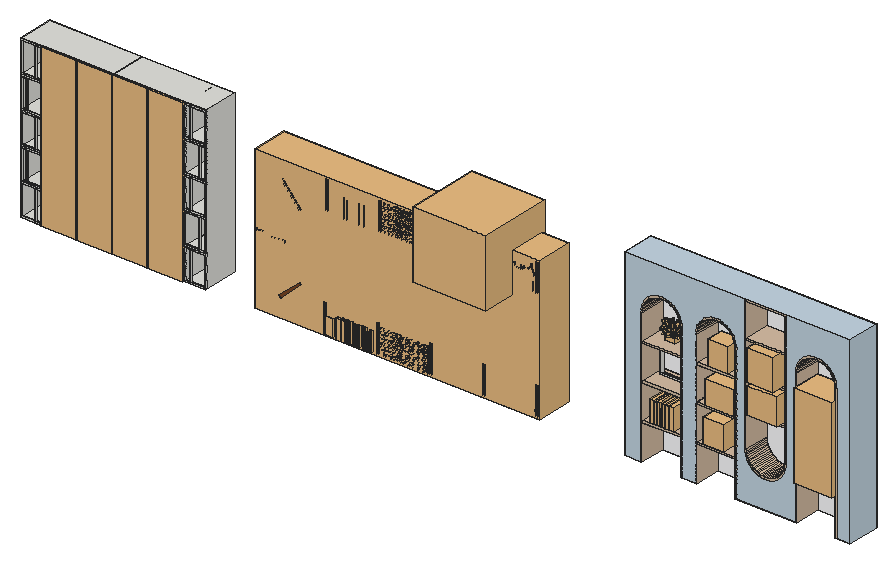
# SketchUp Ruby script. Lengths in millimetres.
U = 1.mm
M = Sketchup.active_model
def pt(a) = Geom::Point3d.new(a.map { |v| v * U })
def face(e, loops, mat)
  f = e.add_face(loops[0].map { |a| pt(a) })
  loops[1..].each { |l| e.add_face(l.map { |a| pt(a) }).erase! }
  f.material = f.back_material = mat if mat
  f
end
# faces: each face lists its corners as indices into pts; further lists are holes
def faces(e, pts, list, mat = nil) = list.each { |f| face(e, (f[0].is_a?(Array) ? f : [f]).map { |l| l.map { |i| pts[i] } }, mat) }
# xy, xz, yz: faces in a plane at the given z, y or x. An outline is a flat list of corners, or four numbers for a rectangle; further outlines are holes
def ring(l) = l.size == 4 ? [[l[0], l[1]], [l[2], l[1]], [l[2], l[3]], [l[0], l[3]]] : l.each_slice(2).to_a
def flat(e, list, mat, &to3) = list.each { |f| face(e, (f[0].is_a?(Array) ? f : [f]).map { |l| ring(l).map { |u, v| to3.(u, v) } }, mat) }
def xy(e, z, list, mat = nil) = flat(e, list, mat) { |x, y| [x, y, z] }
def xz(e, y, list, mat = nil) = flat(e, list, mat) { |x, z| [x, y, z] }
def yz(e, x, list, mat = nil) = flat(e, list, mat) { |y, z| [x, y, z] }
def lines(e, pts, list) = list.each { |a, b| e.add_line(pt(pts[a]), pt(pts[b])) }
# prism: a flat outline (further loops are holes) pulled along v
def prism(e, loops, v, mat = nil)
  f = face(e, loops, mat); d = Geom::Vector3d.new(v.map { |x| x * U })
  f.pushpull(f.normal.samedirection?(d) ? d.length : -d.length)
end
def box(e, o, s, mat = nil) = prism(e, [[o, [o[0] + s[0], o[1], o[2]], [o[0] + s[0], o[1] + s[1], o[2]], [o[0], o[1] + s[1], o[2]]]], [0, 0, s[2]], mat)
def at(x, y, z, deg = 0) = Geom::Transformation.translation(pt([x, y, z])) * Geom::Transformation.rotation(ORIGIN, Z_AXIS, deg.degrees)
def axes(o, x, y, z) = Geom::Transformation.new([*x, 0, *y, 0, *z, 0, *pt(o).to_a, 1])
def part(name) = M.definitions.add(name)
# library, detail: a bought-in or finely detailed component or shape, given as its bounding box
def library(name, o, s) = part(name).tap { |d| box(d.entities, o, s) }
def detail(e, o, s) = box(e.add_group.entities, o, s)
def put(e, d, t, mat = nil) = e.add_instance(d, t).tap { |i| i.material = mat if mat }
def group(e, t, mat = nil) = e.add_group.tap { |g| g.transformation = t; g.material = mat if mat }.entities
root = M.entities
M.materials.add("Material~26").color = [121, 120, 117]
M.materials.add("Material~27").color = [130, 129, 127]
M.materials.add("Material~28").color = [131, 130, 129]
M.materials.add("Material~29").color = [119, 120, 115]
M.materials.add("Material~30").color = [120, 117, 114]
M.materials.add("Material~31").color = [121, 119, 117]
M.materials.add("Material~32").color = [21, 20, 18]
M.materials.add("Material~33").color = [25, 25, 23]
M.materials.add("Material~34").color = [109, 108, 106]
M.materials.add("Material~35").color = [120, 119, 118]
M.materials.add("Material~36").color = [34, 33, 33]
M.materials.add("Material~37").color = [104, 103, 91]
M.materials.add("Material~38").color = [106, 95, 72]
M.materials.add("Material~39").color = [33, 29, 24]
M.materials.add("Material~40").color = [127, 124, 119]
M.materials.add("Material~41").color = [118, 115, 112]
M.materials.add("Material~42").color = [32, 34, 33]
M.materials.add("Material~43").color = [40, 35, 29]
M.materials.add("Material~44").color = [125, 125, 122]
M.materials.add("Material~45").color = [118, 122, 122]
M.materials.add("Material~46").color = [30, 29, 26]
M.materials.add("Material~47").color = [27, 28, 21]
M.materials.add("Material~48").color = [21, 20, 18]
M.materials.add("Material~49").color = [127, 124, 121]
M.materials.add("Material~50").color = [128, 121, 110]
M.materials.add("Material~51").color = [124, 124, 122]
M.materials.add("Material~52").color = [71, 70, 67]
M.materials.add("Material~53").color = [25, 26, 25]
M.materials.add("Material~54").color = [122, 115, 107]
M.materials.add("Material~55").color = [102, 101, 100]
M.materials.add("Material~56").color = [120, 119, 118]
M.materials.add("Material~57").color = [109, 108, 106]
M.materials.add("Material~58").color = [104, 103, 91]
M.materials.add("Material~59").color = [106, 95, 72]
M.materials.add("PDM_Timber_01").color = [134, 117, 87]
M.materials.add("[Blinds_Vertical_Stripe_Gray]").color = [159, 159, 159]
M.materials.add("[Color M09]").color = [0, 0, 0]
M.materials.add("[Color_001]").color = [226, 226, 226]
M.materials.add("[Color_006]").color = [86, 86, 86]
M.materials.add("[Color_A05]").color = [255, 204, 204]
M.materials.add("[Color_A19]").color = [102, 61, 61]
M.materials.add("[Color_A20]").color = [102, 81, 81]
M.materials.add("[Color_B03]").color = [255, 140, 101]
M.materials.add("[Color_B04]").color = [255, 178, 153]
M.materials.add("[Color_B05]").color = [255, 216, 204]
M.materials.add("[Color_C05]").color = [255, 229, 204]
M.materials.add("[Color_C15]").color = [153, 137, 122]
M.materials.add("[Color_D05]").color = [255, 242, 204]
M.materials.add("[Color_D10]").color = [204, 193, 163]
M.materials.add("[Color_D20]").color = [102, 96, 81]
M.materials.add("[Color_E04]").color = [255, 255, 153]
M.materials.add("[Color_E05]").color = [255, 255, 204]
M.materials.add("[Color_E18]").color = [102, 102, 40]
M.materials.add("[Color_G15]").color = [122, 153, 122]
M.materials.add("[Color_I10]").color = [163, 163, 204]
M.materials.add("[Color_I13]").color = [61, 61, 153]
M.materials.add("[Color_I22]").color = [10, 10, 51]
M.materials.add("[Color_L04]").color = [255, 153, 204]
M.materials.add("[Formica Laminate Light]").color = [213, 189, 164]
M.materials.add("[Metal_Brass_Ceiling]").color = [125, 102, 93]
M.materials.add("[Polished Concrete New]").color = [168, 168, 168]
M.materials.add("[Quartz Light Grey]").color = [251, 251, 252]
M.materials.add("[Terrazzo Light Blue]").color = [196, 214, 227]
M.materials.add("[Wood Veneer 01]").color = [120, 70, 37]
c1 = part("Rectangular frame")
prism(c1.entities,[[[300,0,450],[0,0,450],[0,0,0],[300,0,0]],[[284,0,16],[99.2,0,16],[99.2,0,434],[284,0,434]],[[80.7,0,434],[80.7,0,16],[16,0,16],[16,0,434]]],[0,16,0])
c2 = part("Joinery panel")
box(c2.entities,[0,0,0],[30,500,390])
c3 = part("Row of books \#2")
xy(c3.entities,211.6,[[0,541.4,180.2,552.7]],"[Color_D05]")
xy(c3.entities,221.1,[[0,502,180.2,541.4]],"[Color_L04]")
xy(c3.entities,226,[[0,211.2,180.2,238.8]],"[Color_A20]")
xy(c3.entities,226,[[0,179,180.2,194.7]],"[Color_E05]")
xy(c3.entities,229.1,[[0,146.8,180.2,158.7],[0,194.7,180.2,211.2]],"[Color_I10]")
xy(c3.entities,230.9,[[0,552.7,180.2,581.8]],"[Color_C05]")
xy(c3.entities,239.2,[[0,238.8,180.2,259.8]],"[Color_B03]")
xy(c3.entities,246.4,[[0,0,180.2,14.4]],"[Color_I13]")
xy(c3.entities,247,[[0,115.8,180.2,122.7]],"[Color_A05]")
xy(c3.entities,257.4,[[0,438.1,180.2,454.4]],"[Color_C05]")
xy(c3.entities,259.7,[[0,489.2,180.2,502]],"[Color_E18]")
xy(c3.entities,262,[[0,122.7,180.2,132.4]],"[Color_A05]")
xy(c3.entities,262.3,[[0,72.3,180.2,83.9]],"[Color_B05]")
xy(c3.entities,267.7,[[0,278.8,180.2,301.7]],"[Color_006]")
xy(c3.entities,274.4,[[0,104.2,180.2,115.8]],"[Color_001]")
xy(c3.entities,274.4,[[0,83.9,180.2,104.2]],"[Color_A19]")
xy(c3.entities,274.9,[[0,158.7,180.2,179]],"[Color_D05]")
xy(c3.entities,275.5,[[0,395.3,180.2,438.1]],"[Color_B05]")
xy(c3.entities,275.5,[[0,339.9,180.2,357.7]],"[Color_D10]")
xy(c3.entities,275.5,[[0,259.8,180.2,278.8]],"[Color_E05]")
xy(c3.entities,277.8,[[0,14.4,180.2,23.5]],"[Color_E05]")
xy(c3.entities,278.7,[[0,301.7,180.2,315.8]],"[Color_B04]")
xy(c3.entities,278.7,[[0,357.7,180.2,375.2]],"[Color_E04]")
xy(c3.entities,282.4,[[0,59.1,180.2,72.3]],"[Color_B05]")
xy(c3.entities,283.3,[[0,315.8,180.2,339.9]],"[Color_006]")
xy(c3.entities,283.3,[[0,375.2,180.2,395.3]],"[Color_C15]")
xy(c3.entities,298.5,[[0,132.4,180.2,146.8]],"[Color_E05]")
xy(c3.entities,300,[[0,44.1,180.2,59.1]],"[Color_G15]")
xy(c3.entities,304,[[0,454.4,180.2,466.9]],"[Color_C05]")
xy(c3.entities,332.2,[[0,466.9,180.2,489.2]],"[Color_C05]")
xy(c3.entities,342,[[0,23.5,180.2,44.1]],"[Color_006]")
xz(c3.entities,14.4,[[0,246.4,180.2,277.8]],"[Color_E05]")
xz(c3.entities,23.5,[[0,277.8,180.2,342]],"[Color_D20]")
xz(c3.entities,44.1,[[0,300,180.2,342]],"[Color_006]")
xz(c3.entities,59.1,[[0,282.4,180.2,300]],"[Color_G15]")
xz(c3.entities,72.3,[[0,262.3,180.2,282.4]],"[Color_B05]")
xz(c3.entities,83.9,[[0,262.3,180.2,274.4]],"[Metal_Brass_Ceiling]")
xz(c3.entities,115.8,[[0,247,180.2,274.4]],"[Metal_Brass_Ceiling]")
xz(c3.entities,122.7,[[0,247,180.2,262]],"[Metal_Brass_Ceiling]")
xz(c3.entities,132.4,[[0,262,180.2,298.5]],"[Metal_Brass_Ceiling]")
xz(c3.entities,146.8,[[0,229.1,180.2,298.5]],"[Color_E05]")
xz(c3.entities,158.7,[[0,229.1,180.2,274.9]],"[Metal_Brass_Ceiling]")
xz(c3.entities,179,[[0,226,180.2,274.9]],"[Color_D05]")
xz(c3.entities,194.7,[[0,226,180.2,229.1]],"[Metal_Brass_Ceiling]")
xz(c3.entities,211.2,[[0,226,180.2,229.1]],"[Metal_Brass_Ceiling]")
xz(c3.entities,238.8,[[0,226,180.2,239.2]],"[Color_B03]")
xz(c3.entities,259.8,[[0,239.2,180.2,275.5]],"[Color_E05]")
xz(c3.entities,278.8,[[0,267.7,180.2,275.5]],"[Metal_Brass_Ceiling]")
xz(c3.entities,301.7,[[0,267.7,180.2,278.7]],"[Color_B04]")
xz(c3.entities,315.8,[[0,278.7,180.2,283.3]],"[Color_006]")
xz(c3.entities,339.9,[[0,275.5,180.2,283.3]],"[Metal_Brass_Ceiling]")
xz(c3.entities,357.7,[[0,275.5,180.2,278.7]],"[Metal_Brass_Ceiling]")
xz(c3.entities,375.2,[[0,278.7,180.2,283.3]],"[Color_C15]")
xz(c3.entities,395.3,[[0,275.5,180.2,283.3]],"[Metal_Brass_Ceiling]")
xz(c3.entities,438.1,[[0,257.4,180.2,275.5]],"[Metal_Brass_Ceiling]")
xz(c3.entities,454.4,[[0,259.7,180.2,304]],"[Color_C05]")
xz(c3.entities,454.4,[[0,257.4,180.2,259.7]],"[Metal_Brass_Ceiling]")
xz(c3.entities,466.9,[[0,304,180.2,332.2]],"[Color_C05]")
xz(c3.entities,489.2,[[0,259.7,180.2,332.2]],"[Color_C05]")
xz(c3.entities,502,[[0,221.1,180.2,259.7]],"[Color_E18]")
xz(c3.entities,541.4,[[0,211.6,180.2,221.1]],"[Color_L04]")
xz(c3.entities,552.7,[[0,211.6,180.2,230.9]],"[Color_C05]")
xz(c3.entities,581.8,[[0,0,180.2,230.9]],"[Color_C05]")
yz(c3.entities,0,[[581.8,0,14.1,6.3,0,246.4,14.4,246.4,14.4,277.8,23.5,277.8,23.5,342,44.1,342,44.1,300,59.1,300,59.1,282.4,72.3,282.4,72.3,262.3,83.9,262.3,83.9,274.4,115.8,274.4,115.8,247,122.7,247,122.7,262,132.4,262,132.4,298.5,146.8,298.5,146.8,229.1,158.7,229.1,158.7,274.9,179,274.9,179,226,194.7,226,194.7,229.1,211.2,229.1,211.2,226,238.8,226,238.8,239.2,259.8,239.2,259.8,275.5,278.8,275.5,278.8,267.7,301.7,267.7,301.7,278.7,315.8,278.7,315.8,283.3,339.9,283.3,339.9,275.5,357.7,275.5,357.7,278.7,375.2,278.7,375.2,283.3,395.3,283.3,395.3,275.5,438.1,275.5,438.1,257.4,454.4,257.4,454.4,304,466.9,304,466.9,332.2,489.2,332.2,489.2,259.7,502,259.7,502,221.1,541.4,221.1,541.4,211.6,552.7,211.6,552.7,230.9,581.8,230.9]],"[Color_I22]")
yz(c3.entities,180.2,[[581.8,0,581.8,230.9,552.7,230.9,552.7,211.6,541.4,211.6,541.4,221.1,502,221.1,502,259.7,489.2,259.7,489.2,332.2,466.9,332.2,466.9,304,454.4,304,454.4,257.4,438.1,257.4,438.1,275.5,395.3,275.5,395.3,283.3,375.2,283.3,375.2,278.7,357.7,278.7,357.7,275.5,339.9,275.5,339.9,283.3,315.8,283.3,315.8,278.7,301.7,278.7,301.7,267.7,278.8,267.7,278.8,275.5,259.8,275.5,259.8,239.2,238.8,239.2,238.8,226,211.2,226,211.2,229.1,194.7,229.1,194.7,226,179,226,179,274.9,158.7,274.9,158.7,229.1,146.8,229.1,146.8,298.5,132.4,298.5,132.4,262,122.7,262,122.7,247,115.8,247,115.8,274.4,83.9,274.4,83.9,262.3,72.3,262.3,72.3,282.4,59.1,282.4,59.1,300,44.1,300,44.1,342,23.5,342,23.5,277.8,14.4,277.8,14.4,246.4,0,246.4,14.1,6.3]],"[Metal_Brass_Ceiling]")
p = [[0,14.1,6.3],[0,581.8,0],[180.2,581.8,0],[180.2,14.1,6.3],[0,0,246.4],[180.2,0,246.4]]
faces(c3.entities,p,[[0,1,2,3]],"[Color_I22]")
faces(c3.entities,p,[[4,0,3,5]],"[Color_I13]")
c4 = library("Books 1",[183.2,0,0],[416,258,342.5])
c5 = library("Book",[0,0,0],[896.4,282.6,347.1])
c6 = library("3DGeom~26_Defintion",[-11095.2,-10854.4,113.9],[14060.5,21723.9,25400])
c7 = library("3DGeom~27_Defintion",[-14456.9,-9906.2,54.2],[9732.2,17899.1,25400])
c8 = library("3DGeom~28_Defintion",[-17680.6,-9902,24.8],[5190.8,19054.2,25400])
c9 = library("3DGeom~29_Defintion",[-20379.5,-8929,1.3],[3277.7,18917.5,25400])
c10 = library("3DGeom~30_Defintion",[-24221.1,-9153.4,16.2],[3047.4,23119.2,25400])
c11 = library("3DGeom~31_Defintion",[-28800.4,-8127.5,19.8],[2321.6,15955.4,25400])
c12 = library("3DGeom~32_Defintion",[-30038.5,-9335.8,9.8],[3429.2,18196.5,25400])
c13 = library("3DGeom~33_Defintion",[-32428.8,-9649.4,8.7],[3319,22558,25400])
c14 = library("3DGeom~34_Defintion",[-35160.2,-6460.3,-0.7],[2939.8,19260.6,25400])
c15 = library("3DGeom~35_Defintion",[-38473,-8602.2,-0.7],[3296.5,18205.3,25400])
c16 = library("3DGeom~36_Defintion",[-40611.5,-8880.8,18.9],[2391.7,20716.3,25400])
c17 = library("3DGeom~37_Defintion",[-51653.4,-10377.6,4.6],[3568.4,16896.5,25400])
c18 = library("3DGeom~38_Defintion",[-53854.1,-11169.8,13.3],[3252.3,18190.2,25400])
c19 = library("3DGeom~39_Defintion",[-51361.4,-9447.8,-0.6],[2807.7,18911,25400])
c20 = library("3DGeom~56_Defintion",[-9109,-12700,-3305.6],[18205.3,25400,3296.5])
c21 = library("3DGeom~57_Defintion",[-12257.6,-13811.2,2.9],[20144.9,25400,2769.9])
c22 = library("3DGeom~59_Defintion",[-11966.4,-15397.7,6013.7],[20965,25400,2831.4])
c23 = library("3DGeom~44_Defintion",[84.4,-10589,-12992],[3118.1,21192.7,25400])
c24 = library("3DGeom~45_Defintion",[-2729.6,-11738,-14526.8],[2810.7,18895.1,25400])
c25 = library("3DGeom~46_Defintion",[-5947.8,-12336.7,-15007.9],[3111.9,18731.1,25400])
c26 = library("3DGeom~47_Defintion",[-8301.1,-11191.3,-13180.8],[3048.1,20716.4,25400])
c27 = library("3DGeom~48_Defintion",[-11605.7,-11278.1,-13716.4],[2962.5,21381.4,25400])
c28 = library("3DGeom~49_Defintion",[-13295.7,-10615.4,-13054.6],[2238.5,22294.9,25400])
c29 = library("3DGeom~50_Defintion",[-19494.9,-11771.6,-16659],[2526.4,17230.3,25400])
c30 = library("3DGeom~51_Defintion",[-18833.7,-10620.9,-13219.8],[3321.6,22575.5,25400])
c31 = library("3DGeom~52_Defintion",[-22043.6,-11161.6,-13144.4],[3302.9,22448.7,25400])
c32 = library("3DGeom~53_Defintion",[-25823.1,-10667.4,-12917.2],[4158.3,22055.6,25400])
c33 = library("3DGeom~54_Defintion",[-39244.4,-11229.2,-13595.7],[11980.7,23284.2,25400])
c34 = library("3DGeom~55_Defintion",[-54289.9,-12842.8,-16142.4],[16002.9,17654.2,25400])
c35 = library("3DGeom~40_Defintion",[-12133.2,-12691.2,8],[24266.4,25400,2912])
c36 = library("3DGeom~41_Defintion",[-10930.1,-13334.2,2693.7],[25400,23135.4,3003.8])
c37 = library("3DGeom~42_Defintion",[-13045.9,-12788.2,6048.1],[25400,22030.9,2710.9])
c38 = library("3DGeom~43_Defintion",[-10428.8,-13940,8798],[25400,23701.4,2381.4])
c39 = library("3DGeom~58_Defintion",[-6052.8,-16750.4,3473.7],[16896.5,25400,3568.4])
c40 = library("aaa",[7013.9,23346,0],[432.3,438.3,515.7])
c41 = library("Potted trailing plant",[-343.3,-349.2,-188.3],[1030.1,1030.2,947.7])
c42 = part("Group\#1")
xy(c42.entities,0,[[0,0,1300,500]])
xy(c42.entities,16,[[16,0,284,440]])
xy(c42.entities,20,[[320,0,1280,440]])
xy(c42.entities,434,[[16,0,284,440]])
xy(c42.entities,450,[[16,0,284,440]])
xy(c42.entities,884,[[16,0,284,440]])
xy(c42.entities,900,[[16,0,284,440]])
xy(c42.entities,1350,[[16,0,284,440]])
xy(c42.entities,1366,[[16,0,284,440]])
xy(c42.entities,1800,[[16,0,284,440]])
xy(c42.entities,1816,[[16,0,284,440]])
xy(c42.entities,2230,[[320,0,1280,440]])
xy(c42.entities,2234,[[16,0,284,440]])
xy(c42.entities,2250,[[0,0,1300,500]])
xz(c42.entities,0,[[[0,0,300,450],[16,16,284,434]],[[300,0,1300,2250],[320,20,1280,2230]],[0,450,16,884],[284,450,300,884],[0,884,16,900],
  [16,884,284,900],[284,884,300,900],[0,900,16,1350],[284,900,300,1350],[0,1350,300,1350,300,1800,284,1800,284,1366,16,1366,16,1800,0,1800],
  [[0,1800,300,2250],[16,1816,284,2234]]])
xz(c42.entities,440,[[16,16,284,434],[320,20,1280,2230],[16,450,284,884],[16,900,284,1350],[16,1366,284,1800],
  [16,1816,284,2234]])
xz(c42.entities,500,[[0,0,1300,2250]])
yz(c42.entities,0,[[0,0,500,2250]])
yz(c42.entities,16,[[0,16,440,434],[0,450,440,884],[0,900,440,1350],[0,1366,440,1800],[0,1816,440,2234]])
yz(c42.entities,284,[[0,16,440,434],[0,450,440,884],[0,900,440,1350],[0,1366,440,1800],[0,1816,440,2234]])
yz(c42.entities,320,[[0,20,440,450],[0,450,440,884],[0,884,440,900],[0,900,440,1350],[0,1350,440,1800],
  [0,1800,440,2230]])
yz(c42.entities,1280,[[0,20,440,2230]])
yz(c42.entities,1300,[[0,0,500,2250]])
c43 = library("Group\#3",[0,0,0],[505.5,36,2250])
c44 = library("Group\#2",[0,0,0],[505.5,36,2250])
c45 = library("Group\#32",[0,0,0],[505.5,36,2250])
c46 = library("Group\#4",[0,0,0],[4000,510,2000])
c47 = library("DECORATIVE ITEM @ADS",[0,0,0],[481.1,457.9,648.9])
c48 = library("Row of books",[0,0,-2.9],[301,352.1,415.9])
c49 = library("Row of books \#1",[0,0,0],[257.2,197.5,238.3])
c50 = library("组\#2",[0,0,0],[73453,73453,103230])
c51 = library("组\#1",[0,0,0],[36650.3,5469.5,5415.8])
c52 = part("组\#9")
put(c52.entities,c51,axes([1497.7,24394.7,5.5],[1.26228,0.48797,3.25205],[-0.34269,0.93942,-0.00795],[-2.77024,-1.00019,1.22534]),"[Blinds_Vertical_Stripe_Gray]")
put(c52.entities,c51,axes([431.6,24076.6,-100.7],[2.19622,0.01451,1.37277],[-0.00092,0.99996,-0.00909],[-1.69088,0.02303,2.7049]),"[Blinds_Vertical_Stripe_Gray]")
put(c52.entities,c51,axes([-433.8,24189.3,-52.3],[2.00781,-0.76565,2.79101],[0.36701,0.93018,-0.00884],[-2.34501,0.94374,1.94586]),"[Blinds_Vertical_Stripe_Gray]")
c53 = part("组\#10")
put(c53.entities,c52,axes([760,45902,0],[1,0,0],[0,1,0],[0,0,0.62619]))
put(c53.entities,c52,axes([-13547.5,56936.4,0],[0.82314,-0.56784,0],[0.56784,0.82314,0],[0,0,0.62619]))
put(c53.entities,c52,axes([-19876.4,66068.5,47.1],[0.36162,-0.93232,0],[0.93232,0.36162,0],[0,0,0.93928]))
put(c53.entities,c52,at(0,45902,56.2))
c54 = part("组\#11")
p = [[75740.5,82537.8,0],[76210.1,82190,10.6],[80100.6,73763.1,131.3],[78271.1,75091.3,139.1],[75924.4,76795,149.1],[72953.5,78951.9,161.7],
  [82870.3,77257.4,160.3],[70082.3,75271.1,149.3],[78451.6,75424,140.3],[76184.9,77069.7,149.9],[76507.5,77267.6,150.4],[76870.4,77375.2,150.4],
  [77248.8,77385.3,150],[77616.9,77297,149.2],[77949.6,77116.5,148.1],[78224.3,76856.1,146.7],[78422.2,76533.4,145.1],[78529.8,76170.5,143.4],
  [78539.9,75792.1,141.8]]
faces(c54.entities,p,[[0,1,2],[1,2,3,4,5],[6,2,1],[5,4,3,2,7],[8,3,4,9,10,11,12,13,14,15,16,17,18]])
put(c54.entities,c53,at(79294.4,148948.9,0,-180))
put(c54.entities,c53,at(3891.7,79294.4,0,-90))
put(c54.entities,c53,at(73546.2,3891.7,0))
put(c54.entities,c53,at(148948.9,73546.2,0,90))
c55 = part("组\#3")
put(c55.entities,c50,axes([39610.9,38953.8,37162.8],[1,0,0],[0,1,0],[0,0,0.64]))
put(c55.entities,c54,axes([0,0,81245.7],[1,0,0],[0,1,0],[0,0,1.77378]))
c56 = part("planta interior bote blanco pinchos")
put(c56.entities,c55,at(-66694.5,-123958.5,-101393.2))
c57 = part("Group\#6")
box(c57.entities,[0,0,499.7],[534.5,360,30])
box(c57.entities,[0,0,999.5],[534.5,360,30])
box(c57.entities,[0,0,0],[534.5,360,30])
c58 = library("Group\#687",[12683.4,7946.4,2311.6],[420.5,201.7,371.5])
c59 = part("cadre Greenery 1 David & David")
prism(c59.entities,[[[2165.2,747,0],[2165.2,747,1494],[3305.2,747,1494],[3305.2,747,0]],[[2220.1,747,1434.1],[2220.1,747,64.1],[3240.1,747,64.1],[3240.1,747,1434.1]]],[0,-40,0])
c60 = library("Group\#461",[-3844.7,-6676.9,-369.4],[392.1,413.7,1193.9])
p = [[12184.8,-6450.6,-5710],[12210.2,-6450.6,-5710],[12210.2,-6425.2,-5710]]
lines(root,p,[[0,1],[1,2],[2,0]])
put(root,c1,at(0,0,450))
put(root,c1,at(0,0,1350))
put(root,c1,axes([300,0,1800],[-1,0,0],[0,1,0],[0,0,1]))
put(root,c1,axes([300,0,0],[-1,0,0],[0,1,0],[0,0,1]))
put(root,c1,axes([300,0,900],[-1,0,0],[0,1,0],[0,0,1]))
put(root,c1,at(2300,0,0))
put(root,c1,at(2300,0,1800))
put(root,c1,at(2300,0,900))
put(root,c1,axes([2600,0,450],[-1,0,0],[0,1,0],[0,0,1]))
put(root,c1,axes([2600,0,1350],[-1,0,0],[0,1,0],[0,0,1]))
put(root,c2,at(7222.8,16,31.2),"[Wood Veneer 01]")
put(root,c2,at(6480.1,16,31.2),"[Wood Veneer 01]")
put(root,c2,at(5737.3,16,31.2),"[Wood Veneer 01]")
put(root,c2,at(4994.6,16,31.2),"[Wood Veneer 01]")
put(root,c2,at(4251.8,16,31.2),"[Wood Veneer 01]")
put(root,c2,at(7222.8,16,1581.2),"[Wood Veneer 01]")
put(root,c2,at(6487.6,16,1581.2),"[Wood Veneer 01]")
put(root,c2,at(5752.3,16,1581.2),"[Wood Veneer 01]")
put(root,c2,at(5017.1,16,1581.2),"[Wood Veneer 01]")
put(root,c2,at(4281.8,16,1581.2),"[Wood Veneer 01]")
put(root,c2,axes([3621,16,281.7],[0.66818,0,-0.744],[0,1,0],[0.744,0,0.66818]),"[Wood Veneer 01]")
put(root,c2,axes([3314.2,16,1019.4],[-0.06748,0,-0.99772],[0,1,0],[0.99772,0,-0.06748]),"[Wood Veneer 01]")
put(root,c2,axes([3906.8,16,1442],[0.7632,0,0.64616],[0,1,0],[-0.64616,0,0.7632]),"[Wood Veneer 01]")
put(root,c3,axes([7191.2,196.2,1579.3],[0,-0.99994,0.01102],[-0.99994,0.00012,0.01102],[0.01102,0.01102,0.99988]))
put(root,c4,axes([4733.7,16,1581.3],[1.7,0,0],[0,1,0],[0,0,1.13858]))
put(root,c5,axes([5024.6,16,31.2],[0.77,0,0],[0,1,0],[0,0,1]))
put(root,c6,axes([4469.3,146.7,28],[-0.00898,0,0],[0,0.01538,0],[0,0,0.01065]),"Material~26")
put(root,c7,axes([4469.3,146.7,28],[-0.00933,0,0],[0,0.01598,0],[0,0,0.01107]),"Material~27")
put(root,c8,axes([4469.3,146.7,28],[-0.00912,0,0],[0,0.01563,0],[0,0,0.01083]),"Material~28")
put(root,c9,axes([4469.3,146.7,28],[-0.00943,0,0],[0,0.01616,0],[0,0,0.01119]),"Material~29")
put(root,c10,axes([4469.3,146.7,28],[-0.00909,0,0],[0,0.01557,0],[0,0,0.01079]),"Material~30")
put(root,c11,axes([4469.3,146.7,28],[-0.00832,0,0],[0,0.01425,0],[0,0,0.00987]),"Material~31")
put(root,c12,axes([4469.3,146.7,28],[-0.00901,0,0],[0,0.01545,0],[0,0,0.0107]),"Material~32")
put(root,c13,axes([4469.3,146.7,28],[-0.00931,0,0],[0,0.01596,0],[0,0,0.01106]),"Material~33")
put(root,c14,axes([4469.3,146.7,28],[-0.00938,0,0],[0,0.01607,0],[0,0,0.01113]),"Material~34")
put(root,c15,axes([4469.3,146.7,28],[-0.00938,0,0],[0,0.01607,0],[0,0,0.01113]),"Material~35")
put(root,c16,axes([4469.3,146.7,28],[-0.00944,0,0],[0,0.01618,0],[0,0,0.01121]),"Material~36")
put(root,c17,axes([4469.3,146.7,28],[-0.00798,0,0],[0,0.01367,0],[0,0,0.00947]),"Material~37")
put(root,c18,axes([4469.3,146.7,28],[-0.00815,0,0],[0,0.01397,0],[0,0,0.00968]),"Material~38")
put(root,c19,axes([4469.3,146.7,28],[-0.00905,0,0],[0,0.0155,0],[0,0,0.01074]),"Material~39")
put(root,c20,axes([3527.5,206.2,1041.7],[0.00008,-0.01349,0.00134],[0.01133,0.00001,-0.00113],[0.00049,0.00049,0.01065]),"Material~56")
put(root,c21,axes([3527.5,206.2,1041.7],[0.00008,-0.01432,0.00142],[0.01203,0.00002,-0.0012],[0.00052,0.00052,0.01131]),"Material~57")
put(root,c22,axes([3527.5,206.2,1041.7],[0.00008,-0.01347,0.00133],[0.01132,0.00001,-0.00112],[0.00049,0.00049,0.01064]),"Material~59")
put(root,c23,axes([4393.5,180.7,1701.6],[-0.01579,0,0],[0,0.01405,0],[0,0,0.01175]),"Material~44")
put(root,c24,axes([4393.5,180.7,1701.6],[-0.01413,0,0],[0,0.01258,0],[0,0,0.01052]),"Material~45")
put(root,c25,axes([4393.5,180.7,1701.6],[-0.01368,0,0],[0,0.01217,0],[0,0,0.01018]),"Material~46")
put(root,c26,axes([4393.5,180.7,1701.6],[-0.01557,0,0],[0,0.01386,0],[0,0,0.01159]),"Material~47")
put(root,c27,axes([4393.5,180.7,1701.6],[-0.01498,0,0],[0,0.01333,0],[0,0,0.01115]),"Material~48")
put(root,c28,axes([4393.5,180.7,1701.6],[-0.01573,0,0],[0,0.014,0],[0,0,0.01171]),"Material~49")
put(root,c29,axes([4393.5,180.7,1701.6],[-0.01233,0,0],[0,0.01098,0],[0,0,0.00918]),"Material~50")
put(root,c30,axes([4393.5,180.7,1701.6],[-0.01553,0,0],[0,0.01383,0],[0,0,0.01156]),"Material~51")
put(root,c31,axes([4393.5,180.7,1701.6],[-0.01562,0,0],[0,0.0139,0],[0,0,0.01163]),"Material~52")
put(root,c32,axes([4393.5,180.7,1701.6],[-0.0159,0,0],[0,0.01415,0],[0,0,0.01183]),"Material~53")
put(root,c33,axes([4393.5,180.7,1701.6],[-0.01506,0,0],[0,0.0134,0],[0,0,0.01121]),"Material~54")
put(root,c34,axes([3981.8,164,174.4],[-0.00761,0,0],[0,0.01303,0],[0,0,0.00903]),"Material~55")
put(root,c35,axes([6956.8,233.3,31.1],[-0.02102,0,0],[0,0.01397,0],[0,0,0.01517]),"Material~40")
put(root,c36,axes([6956.8,233.3,31.1],[-0.02282,0,0],[0,0.01517,0],[0,0,0.01647]),"Material~41")
put(root,c37,axes([6956.8,233.3,31.1],[-0.02153,0,0],[0,0.01432,0],[0,0,0.01554]),"Material~42")
put(root,c38,axes([6956.8,233.3,31.1],[-0.02146,0,0],[0,0.01426,0],[0,0,0.01548]),"Material~43")
put(root,c39,axes([3527.5,206.2,1041.7],[0.00007,-0.01148,0.00114],[0.00964,0.00001,-0.00096],[0.00042,0.00042,0.00906]),"Material~58")
put(root,c40,at(-236.4,-23248.1,422))
put(root,c40,at(-2527.6,-23248.1,422))
put(root,c41,at(6205.8,-89.5,1618.4))
put(root,c42,at(0,16,0))
put(root,c43,at(794.5,-20,0),"[Color M09]")
put(root,c44,axes([805.5,-20,2250],[-1,0,0],[0,1,0],[0,0,-1]),"[Color M09]")
put(root,c45,axes([1794.5,-20,2250],[1,0,0],[0,1,0],[0,0,-1]),"[Color M09]")
put(root,c43,axes([1805.5,-20,0],[-1,0,0],[0,1,0],[0,0,1]),"[Color M09]")
put(root,c42,axes([2600,16,0],[-1,0,0],[0,1,0],[0,0,1]))
put(root,c46,at(3282.8,16,1.2),"[Wood Veneer 01]")
g1 = group(root,at(8469.1,-124,-27.7))
put(g1,c47,axes([1831.4,0,1620.6],[0.75,0,0],[0,1,0],[0,0,0.66315]))
put(g1,c30,axes([271.3,304.7,680.3],[-0.01553,0,0],[0,0.01383,0],[0,0,0.01156]),"Material~51")
put(g1,c28,axes([271.3,304.7,680.3],[-0.01573,0,0],[0,0.014,0],[0,0,0.01171]),"Material~49")
put(g1,c27,axes([271.3,304.7,680.3],[-0.01498,0,0],[0,0.01333,0],[0,0,0.01115]),"Material~48")
put(g1,c26,axes([271.3,304.7,680.3],[-0.01557,0,0],[0,0.01386,0],[0,0,0.01159]),"Material~47")
put(g1,c32,axes([271.3,304.7,680.3],[-0.0159,0,0],[0,0.01415,0],[0,0,0.01183]),"Material~53")
put(g1,c48,axes([1105.4,140,530],[0.94506,0,0],[0,0.69207,0],[0,0,0.81664]))
put(g1,c48,axes([1167.2,140,1531.8],[0.94506,0,0],[0,0.69207,0],[0,0,0.81664]))
put(g1,c49,axes([1537.4,138.6,1025.7],[-1.60179,0,0],[0,1.173,0],[0,0,1.38414]))
put(g1,c29,axes([271.3,304.7,680.3],[-0.01233,0,0],[0,0.01098,0],[0,0,0.00918]),"Material~50")
put(g1,c31,axes([271.3,304.7,680.3],[-0.01562,0,0],[0,0.0139,0],[0,0,0.01163]),"Material~52")
put(g1,c56,axes([489.2,420.3,1590.1],[0.00198,0,0],[0,0.00145,0],[0,0,0.00094]))
put(g1,c57,at(2421.9,140,500),"[Formica Laminate Light]")
put(g1,c57,at(1021.9,140,500),"[Formica Laminate Light]")
put(g1,c58,at(-10901.3,-7878,-1149),"[Polished Concrete New]")
g2 = group(g1,at(2553,328.3,1029.7))
prism(g2,[[[0,0,351],[0,0,0.6],[255.8,0,0.6],[255.8,0,351]],[[12.3,0,15.7],[12.3,0,336.9],[241.2,0,336.9],[241.2,0,15.7]]],[0,40,0])
g3 = group(g1,at(318.1,369.4,1029.7))
put(g3,c59,axes([-669.9,-707,0],[0.3094,0,0],[0,1,0],[0,0,0.28]))
put(g1,c60,axes([7672.1,6763.2,893],[1.36555,0,0],[0,1,0],[0,0,1]),"PDM_Timber_01")
g4 = group(g1,at(0,140,0),"[Terrazzo Light Blue]")
xy(g4,0,[[0,0,0,460,3170,460,3170,0,2956.5,0,2956.5,360,2421.9,360,2421.9,0,1556.5,0,1556.5,360,1021.9,360,1021.9,0,786.5,0,786.5,360,251.9,360,251.9,0]])
xy(g4,1132.6,[[1711.9,0,2246.4,360]],"[Formica Laminate Light]")
xy(g4,1162.6,[[1711.9,0,2246.4,360]],"[Formica Laminate Light]")
xy(g4,1591.7,[[1711.9,0,2246.4,360]],"[Formica Laminate Light]")
xy(g4,1621.7,[[1711.9,0,2246.4,360]],"[Formica Laminate Light]")
xy(g4,2050.9,[[1711.9,0,2246.4,360]],"[Formica Laminate Light]")
xy(g4,2080.9,[[1711.9,0,2246.4,360]],"[Formica Laminate Light]")
xy(g4,2540,[[1711.9,0,2246.4,360]])
xy(g4,2560,[[0,0,3170,460]])
xz(g4,0,[[0,0,231.9,0,231.9,1882.7,232.8,1905.2,235.5,1927.6,239.9,1949.8,246,1971.5,253.8,1992.6,263.3,2013.1,274.3,2032.8,286.8,2051.6,300.8,2069.3,316.1,2085.8,332.7,2101.2,350.4,2115.1,369.1,2127.6,388.8,2138.7,409.3,2148.1,430.4,2155.9,452.2,2162,474.3,2166.4,496.7,2169.1,519.2,2170,541.8,2169.1,564.2,2166.4,586.3,2162,608,2155.9,629.2,2148.1,649.6,2138.7,669.3,2127.6,688.1,2115.1,705.8,2101.2,722.4,2085.8,737.7,2069.3,751.6,2051.6,764.2,2032.8,775.2,2013.1,784.6,1992.6,792.4,1971.5,798.6,1949.8,803,1927.6,805.6,1905.2,806.5,1882.7,806.5,0,1001.9,0,1001.9,1882.7,1002.8,1905.2,1005.5,1927.6,1009.9,1949.8,1016,1971.5,1023.8,1992.6,1033.3,2013.1,1044.3,2032.8,1056.8,2051.6,1070.8,2069.3,1086.1,2085.8,1102.7,2101.2,1120.4,2115.1,1139.1,2127.6,1158.8,2138.7,1179.3,2148.1,1200.4,2155.9,1222.2,2162,1244.3,2166.4,1266.7,2169.1,1289.2,2170,1311.8,2169.1,1334.2,2166.4,1356.3,2162,1378,2155.9,1399.2,2148.1,1419.6,2138.7,1439.3,2127.6,1458.1,2115.1,1475.8,2101.2,1492.4,2085.8,1507.7,2069.3,1521.6,2051.6,1534.2,2032.8,1545.2,2013.1,1554.6,1992.6,1562.4,1971.5,1568.6,1949.8,1573,1927.6,1575.6,1905.2,1576.5,1882.7,1576.5,0,2401.9,0,2401.9,1882.7,2402.8,1905.2,2405.5,1927.6,2409.9,1949.8,2416,1971.5,2423.8,1992.6,2433.3,2013.1,2444.3,2032.8,2456.8,2051.6,2470.8,2069.3,2486.1,2085.8,2502.7,2101.2,2520.4,2115.1,2539.1,2127.6,2558.8,2138.7,2579.3,2148.1,2600.4,2155.9,2622.2,2162,2644.3,2166.4,2666.7,2169.1,2689.2,2170,2711.8,2169.1,2734.2,2166.4,2756.3,2162,2778,2155.9,2799.2,2148.1,2819.6,2138.7,2839.3,2127.6,2858.1,2115.1,2875.8,2101.2,2892.4,2085.8,2907.7,2069.3,2921.6,2051.6,2934.2,2032.8,2945.2,2013.1,2954.6,1992.6,2962.4,1971.5,2968.6,1949.8,2973,1927.6,2975.6,1905.2,2976.5,1882.7,2976.5,0,3170,0,3170,2560,2266.4,2560,2266.4,677.3,2265.5,654.8,2262.9,632.4,2258.5,610.2,2252.4,588.5,2244.6,567.4,2235.1,546.9,2224.1,527.2,2211.6,508.4,2197.6,490.7,2182.3,474.2,2165.7,458.8,2148,444.9,2129.3,432.4,2109.6,421.3,2089.1,411.9,2067.9,404.1,2046.2,398,2024.1,393.6,2001.7,390.9,1979.2,390,1956.6,390.9,1934.2,393.6,1912.1,398,1890.4,404.1,1869.2,411.9,1848.7,421.3,1829.1,432.4,1810.3,444.9,1792.6,458.8,1776,474.2,1760.7,490.7,1746.7,508.4,1734.2,527.2,1723.2,546.9,1713.8,567.4,1705.9,588.5,1699.8,610.2,1695.4,632.4,1692.8,654.8,1691.9,677.3,1691.9,2560,0,2560]])
xz(g4,0,[[231.9,0,251.9,0,251.9,1882.7,252.8,1903.7,255.2,1924.5,259.3,1945.1,265,1965.3,272.3,1985,281.1,2004,291.3,2022.4,303,2039.8,316,2056.3,330.2,2071.7,345.6,2085.9,362.1,2098.9,379.6,2110.6,397.9,2120.8,416.9,2129.6,436.6,2136.9,456.8,2142.6,477.4,2146.7,498.3,2149.2,519.2,2150,540.2,2149.2,561,2146.7,581.6,2142.6,601.8,2136.9,621.5,2129.6,640.6,2120.8,658.9,2110.6,676.3,2098.9,692.8,2085.9,708.2,2071.7,722.5,2056.3,735.5,2039.8,747.1,2022.4,757.4,2004,766.2,1985,773.4,1965.3,779.1,1945.1,783.2,1924.5,785.7,1903.7,786.5,1882.7,786.5,0,806.5,0,806.5,1882.7,805.6,1905.2,803,1927.6,798.6,1949.8,792.4,1971.5,784.6,1992.6,775.2,2013.1,764.2,2032.8,751.6,2051.6,737.7,2069.3,722.4,2085.8,705.8,2101.2,688.1,2115.1,669.3,2127.6,649.6,2138.7,629.2,2148.1,608,2155.9,586.3,2162,564.2,2166.4,541.8,2169.1,519.2,2170,496.7,2169.1,474.3,2166.4,452.2,2162,430.4,2155.9,409.3,2148.1,388.8,2138.7,369.1,2127.6,350.4,2115.1,332.7,2101.2,316.1,2085.8,300.8,2069.3,286.8,2051.6,274.3,2032.8,263.3,2013.1,253.8,1992.6,246,1971.5,239.9,1949.8,235.5,1927.6,232.8,1905.2,231.9,1882.7],[1001.9,0,1021.9,0,1021.9,1882.7,1022.8,1903.7,1025.2,1924.5,1029.3,1945.1,1035,1965.3,1042.3,1985,1051.1,2004,1061.3,2022.4,1073,2039.8,1086,2056.3,1100.2,2071.7,1115.6,2085.9,1132.1,2098.9,1149.6,2110.6,1167.9,2120.8,1186.9,2129.6,1206.6,2136.9,1226.8,2142.6,1247.4,2146.7,1268.3,2149.2,1289.2,2150,1310.2,2149.2,1331,2146.7,1351.6,2142.6,1371.8,2136.9,1391.5,2129.6,1410.6,2120.8,1428.9,2110.6,1446.3,2098.9,1462.8,2085.9,1478.2,2071.7,1492.5,2056.3,1505.5,2039.8,1517.1,2022.4,1527.4,2004,1536.2,1985,1543.4,1965.3,1549.1,1945.1,1553.2,1924.5,1555.7,1903.7,1556.5,1882.7,1556.5,0,1576.5,0,1576.5,1882.7,1575.6,1905.2,1573,1927.6,1568.6,1949.8,1562.4,1971.5,1554.6,1992.6,1545.2,2013.1,1534.2,2032.8,1521.6,2051.6,1507.7,2069.3,1492.4,2085.8,1475.8,2101.2,1458.1,2115.1,1439.3,2127.6,1419.6,2138.7,1399.2,2148.1,1378,2155.9,1356.3,2162,1334.2,2166.4,1311.8,2169.1,1289.2,2170,1266.7,2169.1,1244.3,2166.4,1222.2,2162,1200.4,2155.9,1179.3,2148.1,1158.8,2138.7,1139.1,2127.6,1120.4,2115.1,1102.7,2101.2,1086.1,2085.8,1070.8,2069.3,1056.8,2051.6,1044.3,2032.8,1033.3,2013.1,1023.8,1992.6,1016,1971.5,1009.9,1949.8,1005.5,1927.6,1002.8,1905.2,1001.9,1882.7],[2401.9,0,2421.9,0,2421.9,1882.7,2422.8,1903.7,2425.2,1924.5,2429.3,1945.1,2435,1965.3,2442.3,1985,2451.1,2004,2461.3,2022.4,2473,2039.8,2486,2056.3,2500.2,2071.7,2515.6,2085.9,2532.1,2098.9,2549.6,2110.6,2567.9,2120.8,2586.9,2129.6,2606.6,2136.9,2626.8,2142.6,2647.4,2146.7,2668.3,2149.2,2689.2,2150,2710.2,2149.2,2731,2146.7,2751.6,2142.6,2771.8,2136.9,2791.5,2129.6,2810.6,2120.8,2828.9,2110.6,2846.3,2098.9,2862.8,2085.9,2878.2,2071.7,2892.5,2056.3,2905.5,2039.8,2917.1,2022.4,2927.4,2004,2936.2,1985,2943.4,1965.3,2949.1,1945.1,2953.2,1924.5,2955.7,1903.7,2956.5,1882.7,2956.5,0,2976.5,0,2976.5,1882.7,2975.6,1905.2,2973,1927.6,2968.6,1949.8,2962.4,1971.5,2954.6,1992.6,2945.2,2013.1,2934.2,2032.8,2921.6,2051.6,2907.7,2069.3,2892.4,2085.8,2875.8,2101.2,2858.1,2115.1,2839.3,2127.6,2819.6,2138.7,2799.2,2148.1,2778,2155.9,2756.3,2162,2734.2,2166.4,2711.8,2169.1,2689.2,2170,2666.7,2169.1,2644.3,2166.4,2622.2,2162,2600.4,2155.9,2579.3,2148.1,2558.8,2138.7,2539.1,2127.6,2520.4,2115.1,2502.7,2101.2,2486.1,2085.8,2470.8,2069.3,2456.8,2051.6,2444.3,2032.8,2433.3,2013.1,2423.8,1992.6,2416,1971.5,2409.9,1949.8,2405.5,1927.6,2402.8,1905.2,2401.9,1882.7],[[1979.2,390,2001.7,390.9,2024.1,393.6,2046.2,398,2067.9,404.1,2089.1,411.9,2109.6,421.3,2129.3,432.4,2148,444.9,2165.7,458.8,2182.3,474.2,2197.6,490.7,2211.6,508.4,2224.1,527.2,2235.1,546.9,2244.6,567.4,2252.4,588.5,2258.5,610.2,2262.9,632.4,2265.5,654.8,2266.4,677.3,2266.4,2560,1691.9,2560,1691.9,677.3,1692.8,654.8,1695.4,632.4,1699.8,610.2,1705.9,588.5,1713.8,567.4,1723.2,546.9,1734.2,527.2,1746.7,508.4,1760.7,490.7,1776,474.2,1792.6,458.8,1810.3,444.9,1829.1,432.4,1848.7,421.3,1869.2,411.9,1890.4,404.1,1912.1,398,1934.2,393.6,1956.6,390.9],[1979.2,410,1958.2,410.8,1937.3,413.3,1916.8,417.4,1896.6,423.1,1876.9,430.4,1857.8,439.2,1839.5,449.4,1822.1,461.1,1805.6,474.1,1790.2,488.3,1775.9,503.7,1762.9,520.2,1751.3,537.6,1741,556,1732.2,575,1725,594.7,1719.3,614.9,1715.2,635.5,1712.7,656.3,1711.9,677.3,1711.9,2540,2246.4,2540,2246.4,677.3,2245.6,656.3,2243.1,635.5,2239,614.9,2233.4,594.7,2226.1,575,2217.3,556,2207,537.6,2195.4,520.2,2182.4,503.7,2168.2,488.3,2152.7,474.1,2136.3,461.1,2118.8,449.4,2100.5,439.2,2081.4,430.4,2061.8,423.1,2041.6,417.4,2021,413.3,2000.1,410.8]],[1711.9,1132.6,2246.4,1162.6],
  [1711.9,1591.7,2246.4,1621.7],[1711.9,2050.9,2246.4,2080.9]],"[Formica Laminate Light]")
xz(g4,360,[[251.9,0,786.5,0,786.5,1882.7,785.7,1903.7,783.2,1924.5,779.1,1945.1,773.4,1965.3,766.2,1985,757.4,2004,747.1,2022.4,735.5,2039.8,722.5,2056.3,708.2,2071.7,692.8,2085.9,676.3,2098.9,658.9,2110.6,640.6,2120.8,621.5,2129.6,601.8,2136.9,581.6,2142.6,561,2146.7,540.2,2149.2,519.2,2150,498.3,2149.2,477.4,2146.7,456.8,2142.6,436.6,2136.9,416.9,2129.6,397.9,2120.8,379.6,2110.6,362.1,2098.9,345.6,2085.9,330.2,2071.7,316,2056.3,303,2039.8,291.3,2022.4,281.1,2004,272.3,1985,265,1965.3,259.3,1945.1,255.2,1924.5,252.8,1903.7,251.9,1882.7],[1021.9,0,1556.5,0,1556.5,1882.7,1555.7,1903.7,1553.2,1924.5,1549.1,1945.1,1543.4,1965.3,1536.2,1985,1527.4,2004,1517.1,2022.4,1505.5,2039.8,1492.5,2056.3,1478.2,2071.7,1462.8,2085.9,1446.3,2098.9,1428.9,2110.6,1410.6,2120.8,1391.5,2129.6,1371.8,2136.9,1351.6,2142.6,1331,2146.7,1310.2,2149.2,1289.2,2150,1268.3,2149.2,1247.4,2146.7,1226.8,2142.6,1206.6,2136.9,1186.9,2129.6,1167.9,2120.8,1149.6,2110.6,1132.1,2098.9,1115.6,2085.9,1100.2,2071.7,1086,2056.3,1073,2039.8,1061.3,2022.4,1051.1,2004,1042.3,1985,1035,1965.3,1029.3,1945.1,1025.2,1924.5,1022.8,1903.7,1021.9,1882.7],[2421.9,0,2956.5,0,2956.5,1882.7,2955.7,1903.7,2953.2,1924.5,2949.1,1945.1,2943.4,1965.3,2936.2,1985,2927.4,2004,2917.1,2022.4,2905.5,2039.8,2892.5,2056.3,2878.2,2071.7,2862.8,2085.9,2846.3,2098.9,2828.9,2110.6,2810.6,2120.8,2791.5,2129.6,2771.8,2136.9,2751.6,2142.6,2731,2146.7,2710.2,2149.2,2689.2,2150,2668.3,2149.2,2647.4,2146.7,2626.8,2142.6,2606.6,2136.9,2586.9,2129.6,2567.9,2120.8,2549.6,2110.6,2532.1,2098.9,2515.6,2085.9,2500.2,2071.7,2486,2056.3,2473,2039.8,2461.3,2022.4,2451.1,2004,2442.3,1985,2435,1965.3,2429.3,1945.1,2425.2,1924.5,2422.8,1903.7,2421.9,1882.7],[1979.2,410,2000.1,410.8,2021,413.3,2041.6,417.4,2061.8,423.1,2081.4,430.4,2100.5,439.2,2118.8,449.4,2136.3,461.1,2152.7,474.1,2168.2,488.3,2182.4,503.7,2195.4,520.2,2207,537.6,2217.3,556,2226.1,575,2233.4,594.7,2239,614.9,2243.1,635.5,2245.6,656.3,2246.4,677.3,2246.4,1132.6,1711.9,1132.6,1711.9,677.3,1712.7,656.3,1715.2,635.5,1719.3,614.9,1725,594.7,1732.2,575,1741,556,1751.3,537.6,1762.9,520.2,1775.9,503.7,1790.2,488.3,1805.6,474.1,1822.1,461.1,1839.5,449.4,1857.8,439.2,1876.9,430.4,1896.6,423.1,1916.8,417.4,1937.3,413.3,1958.2,410.8],[1711.9,1132.6,2246.4,1591.7],
  [1711.9,1591.7,2246.4,2050.9],[1711.9,2050.9,2246.4,2540]],"[Quartz Light Grey]")
xz(g4,460,[[0,0,3170,2560]])
yz(g4,0,[[0,0,460,2560]])
yz(g4,251.9,[[0,0,360,1882.7]],"[Formica Laminate Light]")
yz(g4,786.5,[[0,0,360,1882.7]],"[Formica Laminate Light]")
yz(g4,1021.9,[[0,0,360,1882.7]],"[Formica Laminate Light]")
yz(g4,1556.5,[[0,0,360,1882.7]],"[Formica Laminate Light]")
yz(g4,1711.9,[[0,677.3,360,1132.6],[0,1132.6,360,1591.7],[0,1591.7,360,2050.9],[0,2050.9,360,2540]],"[Formica Laminate Light]")
yz(g4,2246.4,[[0,677.3,360,1132.6],[0,1132.6,360,1591.7],[0,1591.7,360,2050.9],[0,2050.9,360,2540]],"[Formica Laminate Light]")
yz(g4,2421.9,[[0,0,360,1882.7]],"[Formica Laminate Light]")
yz(g4,2956.5,[[0,0,360,1882.7]],"[Formica Laminate Light]")
yz(g4,3170,[[0,0,460,2560]])
p = [[1958.2,0,410.8],[1979.2,0,410],[1979.2,360,410],[1958.2,360,410.8],[2000.1,0,410.8],[2000.1,360,410.8],
  [1937.3,0,413.3],[1937.3,360,413.3],[2021,0,413.3],[2021,360,413.3],[1916.8,0,417.4],[1916.8,360,417.4],
  [2041.6,0,417.4],[2041.6,360,417.4],[1896.6,0,423.1],[1896.6,360,423.1],[2061.8,0,423.1],[2061.8,360,423.1],
  [1876.9,0,430.4],[1876.9,360,430.4],[2081.4,0,430.4],[2081.4,360,430.4],[1857.8,0,439.2],[1857.8,360,439.2],
  [2100.5,0,439.2],[2100.5,360,439.2],[1839.5,0,449.4],[1839.5,360,449.4],[2118.8,0,449.4],[2118.8,360,449.4],
  [1822.1,0,461.1],[1822.1,360,461.1],[2136.3,0,461.1],[2136.3,360,461.1],[1805.6,0,474.1],[1805.6,360,474.1],
  [2152.7,0,474.1],[2152.7,360,474.1],[1790.2,0,488.3],[1790.2,360,488.3],[2168.2,0,488.3],[2168.2,360,488.3],
  [1775.9,0,503.7],[1775.9,360,503.7],[2182.4,0,503.7],[2182.4,360,503.7],[1762.9,0,520.2],[1762.9,360,520.2],
  [2195.4,0,520.2],[2195.4,360,520.2],[1751.3,0,537.6],[1751.3,360,537.6],[2207,0,537.6],[2207,360,537.6],
  [1741,0,556],[1741,360,556],[2217.3,0,556],[2217.3,360,556],[1732.2,0,575],[1732.2,360,575],
  [2226.1,0,575],[2226.1,360,575],[1725,0,594.7],[1725,360,594.7],[2233.4,0,594.7],[2233.4,360,594.7],
  [1719.3,0,614.9],[1719.3,360,614.9],[2239,0,614.9],[2239,360,614.9],[1715.2,0,635.5],[1715.2,360,635.5],
  [2243.1,0,635.5],[2243.1,360,635.5],[1712.7,0,656.3],[1712.7,360,656.3],[2245.6,0,656.3],[2245.6,360,656.3],
  [1711.9,0,677.3],[1711.9,360,677.3],[2246.4,0,677.3],[2246.4,360,677.3],[252.8,0,1903.7],[251.9,0,1882.7],
  [251.9,360,1882.7],[252.8,360,1903.7],[786.5,0,1882.7],[785.7,0,1903.7],[785.7,360,1903.7],[786.5,360,1882.7],
  [1022.8,0,1903.7],[1021.9,0,1882.7],[1021.9,360,1882.7],[1022.8,360,1903.7],[1556.5,0,1882.7],[1555.7,0,1903.7],
  [1555.7,360,1903.7],[1556.5,360,1882.7],[2422.8,0,1903.7],[2421.9,0,1882.7],[2421.9,360,1882.7],[2422.8,360,1903.7],
  [2956.5,0,1882.7],[2955.7,0,1903.7],[2955.7,360,1903.7],[2956.5,360,1882.7],[255.2,0,1924.5],[255.2,360,1924.5],
  [783.2,0,1924.5],[783.2,360,1924.5],[1025.2,0,1924.5],[1025.2,360,1924.5],[1553.2,0,1924.5],[1553.2,360,1924.5],
  [2425.2,0,1924.5],[2425.2,360,1924.5],[2953.2,0,1924.5],[2953.2,360,1924.5],[259.3,0,1945.1],[259.3,360,1945.1],
  [779.1,0,1945.1],[779.1,360,1945.1],[1029.3,0,1945.1],[1029.3,360,1945.1],[1549.1,0,1945.1],[1549.1,360,1945.1],
  [2429.3,0,1945.1],[2429.3,360,1945.1],[2949.1,0,1945.1],[2949.1,360,1945.1],[265,0,1965.3],[265,360,1965.3],
  [773.4,0,1965.3],[773.4,360,1965.3],[1035,0,1965.3],[1035,360,1965.3],[1543.4,0,1965.3],[1543.4,360,1965.3],
  [2435,0,1965.3],[2435,360,1965.3],[2943.4,0,1965.3],[2943.4,360,1965.3],[272.3,0,1985],[272.3,360,1985],
  [766.2,0,1985],[766.2,360,1985],[1042.3,0,1985],[1042.3,360,1985],[1536.2,0,1985],[1536.2,360,1985],
  [2442.3,0,1985],[2442.3,360,1985],[2936.2,0,1985],[2936.2,360,1985],[281.1,0,2004],[281.1,360,2004],
  [757.4,0,2004],[757.4,360,2004],[1051.1,0,2004],[1051.1,360,2004],[1527.4,0,2004],[1527.4,360,2004],
  [2451.1,0,2004],[2451.1,360,2004],[2927.4,0,2004],[2927.4,360,2004],[291.3,0,2022.4],[291.3,360,2022.4],
  [747.1,0,2022.4],[747.1,360,2022.4],[1061.3,0,2022.4],[1061.3,360,2022.4],[1517.1,0,2022.4],[1517.1,360,2022.4],
  [2461.3,0,2022.4],[2461.3,360,2022.4],[2917.1,0,2022.4],[2917.1,360,2022.4],[303,0,2039.8],[303,360,2039.8],
  [735.5,0,2039.8],[735.5,360,2039.8],[1073,0,2039.8],[1073,360,2039.8],[1505.5,0,2039.8],[1505.5,360,2039.8],
  [2473,0,2039.8],[2473,360,2039.8],[2905.5,0,2039.8],[2905.5,360,2039.8],[316,0,2056.3],[316,360,2056.3],
  [722.5,0,2056.3],[722.5,360,2056.3],[1086,0,2056.3],[1086,360,2056.3],[1492.5,0,2056.3],[1492.5,360,2056.3],
  [2486,0,2056.3],[2486,360,2056.3],[2892.5,0,2056.3],[2892.5,360,2056.3],[330.2,0,2071.7],[330.2,360,2071.7],
  [708.2,0,2071.7],[708.2,360,2071.7],[1100.2,0,2071.7],[1100.2,360,2071.7],[1478.2,0,2071.7],[1478.2,360,2071.7],
  [2500.2,0,2071.7],[2500.2,360,2071.7],[2878.2,0,2071.7],[2878.2,360,2071.7],[345.6,0,2085.9],[345.6,360,2085.9],
  [692.8,0,2085.9],[692.8,360,2085.9],[1115.6,0,2085.9],[1115.6,360,2085.9],[1462.8,0,2085.9],[1462.8,360,2085.9],
  [2515.6,0,2085.9],[2515.6,360,2085.9],[2862.8,0,2085.9],[2862.8,360,2085.9],[362.1,0,2098.9],[362.1,360,2098.9],
  [676.3,0,2098.9],[676.3,360,2098.9],[1132.1,0,2098.9],[1132.1,360,2098.9],[1446.3,0,2098.9],[1446.3,360,2098.9],
  [2532.1,0,2098.9],[2532.1,360,2098.9],[2846.3,0,2098.9],[2846.3,360,2098.9],[379.6,0,2110.6],[379.6,360,2110.6],
  [658.9,0,2110.6],[658.9,360,2110.6],[1149.6,0,2110.6],[1149.6,360,2110.6],[1428.9,0,2110.6],[1428.9,360,2110.6],
  [2549.6,0,2110.6],[2549.6,360,2110.6],[2828.9,0,2110.6],[2828.9,360,2110.6],[397.9,0,2120.8],[397.9,360,2120.8],
  [640.6,0,2120.8],[640.6,360,2120.8],[1167.9,0,2120.8],[1167.9,360,2120.8],[1410.6,0,2120.8],[1410.6,360,2120.8],
  [2567.9,0,2120.8],[2567.9,360,2120.8],[2810.6,0,2120.8],[2810.6,360,2120.8],[416.9,0,2129.6],[416.9,360,2129.6],
  [621.5,0,2129.6],[621.5,360,2129.6],[1186.9,0,2129.6],[1186.9,360,2129.6],[1391.5,0,2129.6],[1391.5,360,2129.6],
  [2586.9,0,2129.6],[2586.9,360,2129.6],[2791.5,0,2129.6],[2791.5,360,2129.6],[436.6,0,2136.9],[436.6,360,2136.9],
  [601.8,0,2136.9],[601.8,360,2136.9],[1206.6,0,2136.9],[1206.6,360,2136.9],[1371.8,0,2136.9],[1371.8,360,2136.9],
  [2606.6,0,2136.9],[2606.6,360,2136.9],[2771.8,0,2136.9],[2771.8,360,2136.9],[456.8,0,2142.6],[456.8,360,2142.6],
  [581.6,0,2142.6],[581.6,360,2142.6],[1226.8,0,2142.6],[1226.8,360,2142.6],[1351.6,0,2142.6],[1351.6,360,2142.6],
  [2626.8,0,2142.6],[2626.8,360,2142.6],[2751.6,0,2142.6],[2751.6,360,2142.6],[477.4,0,2146.7],[477.4,360,2146.7],
  [561,0,2146.7],[561,360,2146.7],[1247.4,0,2146.7],[1247.4,360,2146.7],[1331,0,2146.7],[1331,360,2146.7],
  [2647.4,0,2146.7],[2647.4,360,2146.7],[2731,0,2146.7],[2731,360,2146.7],[498.3,0,2149.2],[498.3,360,2149.2],
  [540.2,0,2149.2],[540.2,360,2149.2],[1268.3,0,2149.2],[1268.3,360,2149.2],[1310.2,0,2149.2],[1310.2,360,2149.2],
  [2668.3,0,2149.2],[2668.3,360,2149.2],[2710.2,0,2149.2],[2710.2,360,2149.2],[519.2,0,2150],[519.2,360,2150],
  [1289.2,0,2150],[1289.2,360,2150],[2689.2,0,2150],[2689.2,360,2150]]
faces(g4,p,[[0,1,2,3],[1,4,5,2],[6,0,3,7],[4,8,9,5],[10,6,7,11],[8,12,13,9],[14,10,11,15],[12,16,17,13],
  [18,14,15,19],[16,20,21,17],[22,18,19,23],[20,24,25,21],[26,22,23,27],[24,28,29,25],[30,26,27,31],[28,32,33,29],
  [34,30,31,35],[32,36,37,33],[38,34,35,39],[36,40,41,37],[42,38,39,43],[40,44,45,41],[46,42,43,47],[44,48,49,45],
  [50,46,47,51],[48,52,53,49],[54,50,51,55],[52,56,57,53],[58,54,55,59],[56,60,61,57],[62,58,59,63],[60,64,65,61],
  [66,62,63,67],[64,68,69,65],[70,66,67,71],[68,72,73,69],[74,70,71,75],[72,76,77,73],[78,74,75,79],[76,80,81,77],
  [82,83,84,85],[86,87,88,89],[90,91,92,93],[94,95,96,97],[98,99,100,101],[102,103,104,105],[106,82,85,107],[87,108,109,88],
  [110,90,93,111],[95,112,113,96],[114,98,101,115],[103,116,117,104],[118,106,107,119],[108,120,121,109],[122,110,111,123],[112,124,125,113],
  [126,114,115,127],[116,128,129,117],[130,118,119,131],[120,132,133,121],[134,122,123,135],[124,136,137,125],[138,126,127,139],[128,140,141,129],
  [142,130,131,143],[132,144,145,133],[146,134,135,147],[136,148,149,137],[150,138,139,151],[140,152,153,141],[154,142,143,155],[144,156,157,145],
  [158,146,147,159],[148,160,161,149],[162,150,151,163],[152,164,165,153],[166,154,155,167],[156,168,169,157],[170,158,159,171],[160,172,173,161],
  [174,162,163,175],[164,176,177,165],[178,166,167,179],[168,180,181,169],[182,170,171,183],[172,184,185,173],[186,174,175,187],[176,188,189,177],
  [190,178,179,191],[180,192,193,181],[194,182,183,195],[184,196,197,185],[198,186,187,199],[188,200,201,189],[202,190,191,203],[192,204,205,193],
  [206,194,195,207],[196,208,209,197],[210,198,199,211],[200,212,213,201],[214,202,203,215],[204,216,217,205],[218,206,207,219],[208,220,221,209],
  [222,210,211,223],[212,224,225,213],[226,214,215,227],[216,228,229,217],[230,218,219,231],[220,232,233,221],[234,222,223,235],[224,236,237,225],
  [238,226,227,239],[228,240,241,229],[242,230,231,243],[232,244,245,233],[246,234,235,247],[236,248,249,237],[250,238,239,251],[240,252,253,241],
  [254,242,243,255],[244,256,257,245],[258,246,247,259],[248,260,261,249],[262,250,251,263],[252,264,265,253],[266,254,255,267],[256,268,269,257],
  [270,258,259,271],[260,272,273,261],[274,262,263,275],[264,276,277,265],[278,266,267,279],[268,280,281,269],[282,270,271,283],[272,284,285,273],
  [286,274,275,287],[276,288,289,277],[290,278,279,291],[280,292,293,281],[294,282,283,295],[284,296,297,285],[298,286,287,299],[288,300,301,289],
  [302,290,291,303],[292,304,305,293],[306,294,295,307],[296,308,309,297],[310,298,299,311],[300,312,313,301],[314,302,303,315],[304,316,317,305],
  [318,306,307,319],[308,320,321,309],[322,310,311,323],[312,322,323,313],[324,314,315,325],[316,324,325,317],[326,318,319,327],[320,326,327,321]],"[Formica Laminate Light]")
put(g1,c57,at(251.9,140,500),"[Formica Laminate Light]")
